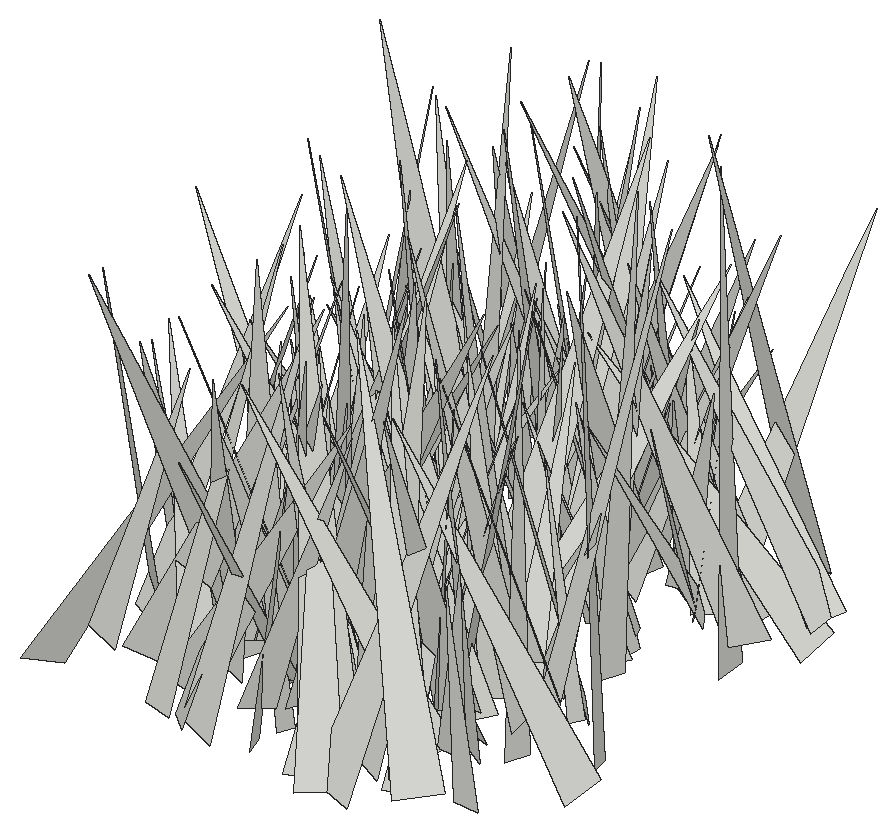
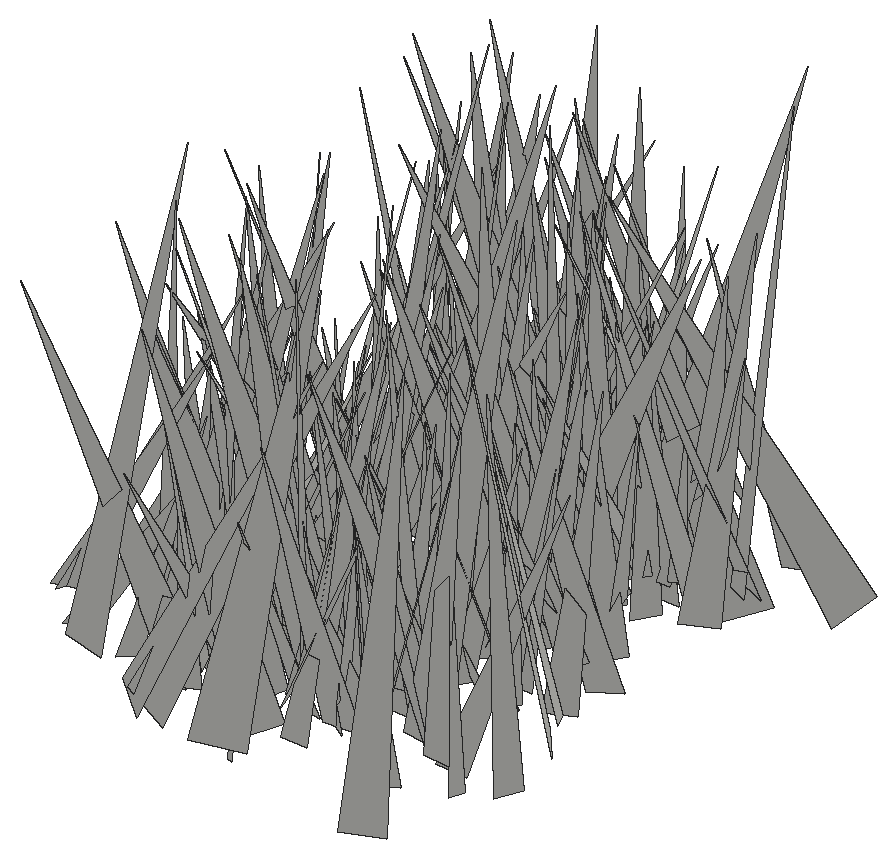
# SketchUp Ruby script. Lengths in inches.
U = 1.inch
M = Sketchup.active_model
def pt(a) = Geom::Point3d.new(a.map { |v| v * U })
def face(e, loops, mat)
  f = e.add_face(loops[0].map { |a| pt(a) })
  loops[1..].each { |l| e.add_face(l.map { |a| pt(a) }).erase! }
  f.material = f.back_material = mat if mat
  f
end
# faces: each face lists its corners as indices into pts; further lists are holes
def faces(e, pts, list, mat = nil) = list.each { |f| face(e, (f[0].is_a?(Array) ? f : [f]).map { |l| l.map { |i| pts[i] } }, mat) }
# xy, xz, yz: faces in a plane at the given z, y or x. An outline is a flat list of corners, or four numbers for a rectangle; further outlines are holes
def ring(l) = l.size == 4 ? [[l[0], l[1]], [l[2], l[1]], [l[2], l[3]], [l[0], l[3]]] : l.each_slice(2).to_a
def flat(e, list, mat, &to3) = list.each { |f| face(e, (f[0].is_a?(Array) ? f : [f]).map { |l| ring(l).map { |u, v| to3.(u, v) } }, mat) }
def xy(e, z, list, mat = nil) = flat(e, list, mat) { |x, y| [x, y, z] }
def xz(e, y, list, mat = nil) = flat(e, list, mat) { |x, z| [x, y, z] }
def yz(e, x, list, mat = nil) = flat(e, list, mat) { |y, z| [x, y, z] }
def lines(e, pts, list) = list.each { |a, b| e.add_line(pt(pts[a]), pt(pts[b])) }
# prism: a flat outline (further loops are holes) pulled along v
def prism(e, loops, v, mat = nil)
  f = face(e, loops, mat); d = Geom::Vector3d.new(v.map { |x| x * U })
  f.pushpull(f.normal.samedirection?(d) ? d.length : -d.length)
end
def box(e, o, s, mat = nil) = prism(e, [[o, [o[0] + s[0], o[1], o[2]], [o[0] + s[0], o[1] + s[1], o[2]], [o[0], o[1] + s[1], o[2]]]], [0, 0, s[2]], mat)
def at(x, y, z, deg = 0) = Geom::Transformation.translation(pt([x, y, z])) * Geom::Transformation.rotation(ORIGIN, Z_AXIS, deg.degrees)
def axes(o, x, y, z) = Geom::Transformation.new([*x, 0, *y, 0, *z, 0, *pt(o).to_a, 1])
def part(name) = M.definitions.add(name)
# library, detail: a bought-in or finely detailed component or shape, given as its bounding box
def library(name, o, s) = part(name).tap { |d| box(d.entities, o, s) }
def detail(e, o, s) = box(e.add_group.entities, o, s)
def put(e, d, t, mat = nil) = e.add_instance(d, t).tap { |i| i.material = mat if mat }
def group(e, t, mat = nil) = e.add_group.tap { |g| g.transformation = t; g.material = mat if mat }.entities
root = M.entities
c1 = part("fur_instance\#9")
p = [[0.8125,0,1.79],[0.67,-0.02,1.48],[0,-0.11,0],[0,0.11,0]]
faces(c1.entities,p,[[0,1,2,3]])
put(root,c1,axes([98.14,124.15,-28.22],[6.1777,-0.38175,1.16241],[-0.13775,-6.16226,-1.29169],[-1.21571,-1.24165,6.0532]))
put(root,c1,axes([98.83,114.34,-27.1],[4.29462,-4.11505,0.26594],[-3.98176,-4.23808,-1.27765],[-1.07236,-0.74374,5.80905]))
put(root,c1,axes([100.36,124.0625,-28.22],[1.56687,-4.2825,0.24372],[-4.04586,-1.5617,-1.43053],[-1.42486,-0.27491,4.32996]))
put(root,c1,axes([99.08,121,-28.22],[5.30824,4.83924,1.79848],[4.88732,-5.54151,0.48577],[-1.6634,-0.83881,7.16657]))
put(root,c1,axes([101.27,111.58,-28.22],[-5.02924,-0.94611,0.83871],[-1.10156,4.96734,-1.00192],[0.62059,1.14984,5.01842]))
put(root,c1,axes([99.2,112.08,-27.1],[-3.9717,-6.10655,1.7462],[-5.81347,4.32471,1.90107],[2.55787,0.34722,7.03209]))
put(root,c1,axes([101.37,114.98,-27.1],[-4.4304,-0.23548,0.66281],[-0.42328,4.26855,-1.31284],[0.56178,1.35914,4.23796]))
put(root,c1,axes([99.04,111.71,-27.1],[3.08355,6.47581,0.56476],[6.50039,-3.07095,-0.27862],[0.00972,-0.62967,7.16706]))
put(root,c1,axes([98.47,121.29,-27.1],[4.57096,2.53062,0.74602],[2.63797,-4.36083,-1.37058],[0.04077,-1.55993,5.04174]))
put(root,c1,axes([98.78,109.9,-27.1],[-0.11529,-4.79427,2.44231],[-5.06003,0.9271,1.58106],[1.8292,2.26244,4.52754]))
put(root,c1,axes([97.04,109.3,-28.22],[7.21653,-2.33327,0.39687],[-2.31249,-6.67999,2.77668],[0.50399,2.75925,7.05779]))
put(root,c1,axes([102.03,123.24,-28.22],[-1.21025,6.4146,1.42422],[6.45546,0.89059,1.47445],[-1.22575,-1.64315,6.35907]))
put(root,c1,axes([99.84,125.43,-27.1],[-1.49561,-5.63035,1.67127],[-5.71638,1.79132,0.91926],[1.34798,1.34949,5.75262]))
put(root,c1,axes([99.95,119.47,-28.22],[3.42227,-3.49613,0.30492],[-3.40506,-3.41104,-0.89344],[-0.84941,-0.41195,4.81005]))
put(root,c1,axes([101.46,111.12,-27.1],[-3.65531,3.57205,1.42816],[3.77376,3.712,0.37448],[0.74692,-1.27356,5.09712]))
put(root,c1,axes([99.32,125.1,-28.22],[4.97524,0.71585,1.07536],[1.04452,-4.74693,-1.67259],[-0.76015,-1.83742,4.74004]))
put(root,c1,axes([99.75,117.6,-28.22],[-0.68675,5.73435,1.62653],[5.78722,1.03346,-1.2],[1.42703,-1.4315,5.64928]))
put(root,c1,axes([101.83,119.48,-28.22],[4.02018,4.80904,4.066],[5.52928,-5.00439,0.45193],[-3.01434,-2.76593,6.25176]))
put(root,c1,axes([102.32,118.93,-28.22],[0.55965,-6.1533,3.26603],[-6.71098,-1.35523,-1.40332],[-1.86889,3.02383,6.01722]))
put(root,c1,axes([99.98,128.72,-28.22],[2.21636,-6.61774,0.25451],[-6.61771,-2.20273,0.35418],[0.25535,0.35358,6.97003]))
put(root,c1,axes([100.23,121.53,-27.1],[3.94789,-1.4658,0.35037],[-1.34081,-3.86465,-1.06014],[-0.68816,-0.87925,4.0756]))
put(root,c1,axes([102.05,125.84,-28.22],[-4.23671,-2.59002,0.97553],[-2.55905,4.34534,0.42292],[1.0541,0.13924,4.94763]))
put(root,c1,axes([99.33,113.69,-27.1],[6.39922,1.66084,0.77373],[1.68967,-6.43637,-0.15871],[-0.70856,-0.34898,6.60932]))
put(root,c1,axes([102.52,122.64,-27.1],[2.49125,-7.31611,3.2771],[-7.62751,-3.2193,-1.38865],[-2.46697,2.5655,7.60286]))
put(root,c1,axes([102.01,113.04,-27.1],[1.8393,-7.94223,0.20343],[-7.82957,-1.84746,-1.33722],[-1.34842,-0.10629,8.04201]))
put(root,c1,axes([104.88,114,-28.22],[-4.31341,6.46311,1.11663],[6.32564,3.74609,2.75266],[-1.73345,-2.41229,7.26637]))
put(root,c1,axes([101.51,119.68,-28.22],[2.15657,3.40289,0.33157],[3.29952,-2.17412,0.8525],[-0.89598,0.18416,3.93747]))
put(root,c1,axes([101.4,117.82,-27.1],[0.40052,6.46259,0.29319],[6.45769,-0.38185,-0.40475],[0.38629,-0.31712,6.46233]))
put(root,c1,axes([101.22,126,-28.22],[1.31397,-3.56018,1.31098],[-3.78942,-1.16427,0.63629],[0.18405,1.44556,3.7412]))
put(root,c1,axes([103.09,118.93,-27.1],[-4.66281,-2.88259,0.04543],[-2.761,4.48988,1.50703],[0.82963,-1.25893,5.27068]))
put(root,c1,axes([102.95,116.25,-27.1],[1.4221,-3.78822,2.5832],[-4.25079,-2.10312,-0.74405],[-1.71882,2.06693,3.97736]))
put(root,c1,axes([101.625,113.34,-28.22],[4.11916,-1.93041,1.42636],[-1.9279,-4.34864,-0.31782],[-1.42975,0.30221,4.53795]))
put(root,c1,axes([100.15,118.57,-27.1],[3.34433,-2.45993,0.06359],[-2.39384,-3.22746,1.0454],[0.56992,0.87868,4.01783]))
put(root,c1,axes([102.38,112.625,-27.1],[4.15865,3.49208,0.81847],[2.77358,-3.92559,2.6563],[-2.27416,1.59814,4.73636]))
put(root,c1,axes([103.42,119.94,-28.22],[-4.44101,1.77663,0.66677],[1.83519,4.45274,0.3588],[0.48276,-0.58331,4.76973]))
put(root,c1,axes([101.59,118.24,-27.1],[3.58428,-2.61771,1.24135],[-2.70899,-3.7283,-0.04015],[-1.02701,0.69843,4.43823]))
put(root,c1,axes([102.42,112.83,-27.1],[-3.32764,3.062,1.30373],[3.08153,3.53122,-0.42827],[1.25687,-0.55083,4.50173]))
put(root,c1,axes([100.88,116,-28.22],[4.9839,-2.53795,0.76874],[-2.53211,-5.04073,-0.2255],[-0.78777,0.14572,5.58834]))
put(root,c1,axes([102,123.35,-27.1],[-0.34341,4.80516,0.97397],[4.88667,0.41477,-0.32328],[0.39826,-0.94579,4.80656]))
put(root,c1,axes([101.98,122.5,-28.22],[7.12046,1.58475,2.39098],[0.70942,-7.17277,2.64146],[-2.77938,2.22916,6.79964]))
put(root,c1,axes([103.02,122.32,-27.1],[2.9733,6.47594,2.08154],[6.51847,-3.36189,1.14821],[-1.94427,-1.36785,7.03277]))
put(root,c1,axes([102.39,119.16,-27.1],[-3.17214,-2.54983,0.51656],[-2.07776,2.97317,1.9168],[1.56569,-1.22048,3.59026]))
put(root,c1,axes([101.21,112.8,-27.1],[0.94954,-6.1364,0.24208],[-6.03443,-0.88683,1.18943],[1.14,0.41683,6.09444]))
put(root,c1,axes([101.74,112.23,-28.22],[-1.04898,-5.12431,2.12616],[-5.35306,1.50327,0.98203],[1.45734,1.83333,5.13756]))
put(root,c1,axes([103.43,113.9,-27.1],[-4.06699,-5.2197,0.56162],[-5.13541,4.10303,0.94539],[1.09007,-0.14467,6.54919]))
put(root,c1,axes([99.42,111.39,-28.22],[4.40599,-6.63506,1.39046],[-6.52465,-3.70025,3.01783],[1.84021,2.76664,7.37085]))
put(root,c1,axes([102.875,113.8125,-28.22],[-5.47966,3.19166,2.7493],[3.39794,6.01513,-0.2105],[2.48986,-1.18473,6.33791]))
put(root,c1,axes([100.78,117.875,-27.1],[6.76067,1.19839,0.69108],[1.18973,-6.79585,0.14582],[-0.7059,0.02372,6.86451]))
put(root,c1,axes([102.77,107.54,-27.1],[3.19327,6.60837,0.52108],[6.51338,-3.23542,1.11669],[-1.23207,0.02336,7.254]))
put(root,c1,axes([102.13,125.58,-28.22],[1.67975,-3.93598,0.16611],[-3.93538,-1.66827,0.26597],[0.17974,0.25696,4.27115]))
put(root,c1,axes([104.22,118.83,-27.1],[-3.8782,-4.63911,2.52217],[-5.26639,3.62608,-1.42825],[0.38461,2.87286,5.87554]))
put(root,c1,axes([102.75,113.11,-28.22],[4.03542,0.28371,1.50858],[-0.2798,-4.0361,1.5075],[-1.50932,1.50677,3.754]))
put(root,c1,axes([105.63,125.09,-27.1],[-6.50715,-2.26194,0.29712],[-2.26712,6.51165,-0.07913],[0.25462,0.17236,6.88863]))
put(root,c1,axes([105.23,110.48,-28.22],[-5.59441,-0.96055,0.72122],[-1.15543,5.24244,-1.98041],[0.32833,2.08191,5.31959]))
put(root,c1,axes([102.46,108.91,-28.22],[4.99959,5.18328,0.38062],[5.01525,-4.9501,1.53324],[-1.36326,0.79826,7.03643]))
put(root,c1,axes([103.625,122.35,-28.22],[0.28904,-4.61969,1.68996],[-4.89331,-0.44312,-0.3744],[-0.50298,1.65624,4.61355]))
put(root,c1,axes([103.96,120.3,-28.22],[-2.34318,3.21724,1.23905],[3.43189,2.31946,0.46753],[0.3286,-1.2829,3.95253]))
put(root,c1,axes([105.48,115.31,-27.1],[-6.50951,0.22142,0.60358],[0.38251,6.26967,1.82536],[0.51674,-1.85181,6.25226]))
put(root,c1,axes([101.25,116.84,-27.1],[4.31446,-3.71791,0.40504],[-3.72385,-4.21342,0.9907],[0.3462,1.01276,5.60856]))
put(root,c1,axes([105.25,120.8,-28.22],[-3.16425,3.77948,0.90882],[3.82647,2.82214,1.58634],[-0.68447,-1.69527,4.66695]))
put(root,c1,axes([103.5,112.99,-27.1],[2.17041,-4.52553,0.56409],[-4.42394,-2.24099,-0.95709],[-1.10786,0.0828,4.92697]))
put(root,c1,axes([103.29,124.42,-28.22],[3.14318,2.78213,1.66083],[2.96777,-3.40061,0.07991],[-1.30037,-1.03624,4.19683]))
put(root,c1,axes([102.6,112.77,-27.1],[4.53182,-5.76132,1.66498],[-5.89155,-4.66684,-0.11276],[-1.12014,1.237,7.32923]))
put(root,c1,axes([102.74,115.75,-27.1],[3.92592,-0.41216,0.89749],[-0.2951,-4.00034,-0.54626],[-0.94248,-0.46433,3.90952]))
put(root,c1,axes([102.89,115.99,-27.1],[7.08469,1.17747,2.52447],[1.61288,-7.35894,-1.094],[-2.27113,-1.55299,7.09806]))
put(root,c1,axes([104.9,114.22,-27.1],[-2.89308,-3.13599,0.85003],[-3.23039,2.89836,-0.3018],[0.34876,0.83187,4.25597]))
put(root,c1,axes([104.75,111.4,-27.1],[-0.95692,-4.60949,0.0097],[-4.59629,0.95343,-0.35816],[-0.34872,0.08227,4.69412]))
put(root,c1,axes([104.39,124.12,-28.22],[-0.48607,6.36101,0.33267],[6.36907,0.48063,0.1158],[-0.09028,-0.34048,6.37851]))
put(root,c1,axes([105.125,125.07,-27.1],[-5.04486,-3.51647,1.75014],[-3.733,5.17856,-0.35556],[1.22196,1.30239,6.1392]))
put(root,c1,axes([103.22,108.76,-28.22],[2.79902,6.82497,1.56007],[7.00009,-2.70115,-0.74237],[0.11309,-1.72399,7.33919]))
put(root,c1,axes([104.97,117.08,-27.1],[4.62611,-3.05223,2.53258],[-2.97331,-5.24406,-0.88892],[-2.62479,0.5609,5.47054]))
put(root,c1,axes([104.53,115.29,-28.22],[-1.51621,-3.26203,0.55212],[-3.23761,1.58793,0.49084],[0.68086,0.28668,3.56354]))
put(root,c1,axes([105.04,125.63,-28.22],[-0.82021,3.34867,1.94688],[3.86928,0.61559,0.57127],[-0.18046,-2.02092,3.4]))
put(root,c1,axes([105.37,124.63,-27.1],[4.87258,-2.82126,2.84071],[-2.53321,-5.63755,-1.25383],[-3.10033,0.17232,5.48903]))
put(root,c1,axes([106.01,112.08,-28.22],[1.80379,6.11401,2.80003],[6.29213,-2.55743,1.53087],[-2.37284,-2.13386,6.18799]))
put(root,c1,axes([104.35,124.18,-27.1],[-6.11732,-3.75265,2.76683],[-3.28898,6.70851,1.82699],[3.3046,-0.26993,6.94018]))
put(root,c1,axes([106.53,121.54,-28.22],[-3.19994,-2.12817,0.10035],[-2.08753,3.09569,-0.91527],[-0.42587,0.81635,3.73243]))
put(root,c1,axes([102.64,116.68,-27.1],[3.58397,-3.64133,0.7361],[-3.60405,-3.15993,1.91614],[0.90107,1.84433,4.7363]))
put(root,c1,axes([102.43,119.9375,-28.22],[2.95433,4.07724,0.35212],[3.82019,-2.59183,-2.04072],[1.46767,-1.46099,4.60298]))
put(root,c1,axes([105.16,119.47,-28.22],[-3.94466,-0.14605,1.57067],[-0.23954,4.23653,-0.20765],[1.55915,0.28136,3.94189]))
put(root,c1,axes([102.15,113.34,-27.1],[0.44147,-7.17503,0.62576],[-6.54369,-0.13768,3.03788],[3.00878,0.75334,6.51516]))
put(root,c1,axes([101.4,110.5625,-28.22],[2.95462,-6.48005,1.02046],[-5.97059,-2.19282,3.36242],[2.71745,2.2277,6.27814]))
put(root,c1,axes([104.05,123.45,-28.22],[4.56042,0.58445,0.815],[0.35248,-4.48653,1.24501],[-0.93891,1.15443,4.42595]))
put(root,c1,axes([103.53,117.95,-28.22],[5.04429,-5.44094,0.7168],[-5.46997,-5.06343,0.05905],[-0.44381,0.56596,7.41924]))
put(root,c1,axes([108.02,115.52,-27.1],[-2.44299,5.49091,1.30941],[5.27932,1.71736,2.64808],[-1.99837,-2.17564,5.395]))
put(root,c1,axes([105.74,124.12,-28.22],[-6.60957,-3.13791,3.29203],[-3.79035,7.01015,-0.92809],[2.51341,2.31982,7.25752]))
put(root,c1,axes([105.08,109.2,-28.22],[3.80415,1.70942,1.42934],[1.7089,-4.05302,0.29902],[-1.42996,-0.29602,4.15984]))
put(root,c1,axes([105.375,128.8,-27.1],[3.52334,-7.25518,1.10129],[-7.15699,-3.66725,-1.26216],[-1.62106,0.42196,7.96608]))
put(root,c1,axes([103.17,113.27,-27.1],[-1.64763,-7.14584,1.34901],[-6.49832,2.06763,3.01567],[3.26416,0.50931,6.68457]))
put(root,c1,axes([104.97,112.11,-28.22],[2.23095,-4.80055,1.901],[-5.14348,-2.24733,0.36107],[-0.45138,1.8816,5.28129]))
put(root,c1,axes([107.02,121.95,-27.1],[0.33091,4.05955,1.18914],[3.81261,-0.80293,1.68011],[-1.83248,-0.93747,3.71034]))
put(root,c1,axes([104.64,122.92,-27.1],[4.0424,-1.6774,0.68877],[-1.67315,-4.09915,-0.16314],[-0.69903,0.11126,4.37357]))
put(root,c1,axes([106.53,111.62,-27.1],[-5.73495,-0.11109,1.68244],[-0.04447,5.97258,0.24275],[1.68552,-0.22038,5.73089]))
put(root,c1,axes([104.8,124.03,-28.22],[4.37398,5.97616,2.1686],[6.29129,-4.44766,-0.43255],[-0.91492,-2.01317,7.39318]))
put(root,c1,axes([105.84,123.94,-28.22],[0.66695,4.37993,0.08385],[4.36286,-0.67176,0.3871],[-0.39533,-0.02429,4.41347]))
put(root,c1,axes([105.49,122.68,-27.1],[4.4988,1.24272,1.44893],[1.33102,-4.70119,-0.10058],[-1.36826,-0.48722,4.6662]))
put(root,c1,axes([104.51,116.63,-27.1],[3.63193,-4.05591,1.60644],[-4.34601,-3.18259,1.79036],[0.37856,2.37544,5.14159]))
put(root,c1,axes([104.67,112.99,-27.1],[1.53942,-5.44162,0.89342],[-5.38829,-1.28703,1.44538],[1.17292,1.22946,5.46735]))
put(root,c1,axes([105.83,127.66,-28.22],[-2.04339,-2.88899,0.9747],[-2.5158,2.26047,1.42575],[1.7225,-0.12566,3.23866]))
put(root,c1,axes([105.66,114.1,-28.22],[4.8037,-2.51399,0.9877],[-2.43404,-4.90267,-0.64073],[-1.17095,-0.12226,5.38379]))
put(root,c1,axes([109.76,126.71,-28.22],[-2.49506,-7.82927,1.12782],[-7.54738,2.00233,-2.79687],[-2.3678,1.86761,7.7266]))
put(root,c1,axes([108.26,124.31,-27.1],[1.91991,5.69676,2.84026],[5.7974,-2.78995,1.67703],[-2.62873,-1.9923,5.77292]))
put(root,c1,axes([103.42,112.56,-28.22],[7.5928,-1.32868,0.07278],[-1.31152,-7.40102,1.71058],[0.22497,1.69728,7.51598]))
put(root,c1,axes([107.43,110.45,-28.22],[0.0044,-6.27087,2.13822],[-6.5778,-0.25997,-0.7489],[-0.79272,2.12236,6.226]))
put(root,c1,axes([107.67,109.45,-27.1],[-5.36752,5.77658,2.45123],[6.12108,5.53013,0.37117],[1.38195,-2.05828,7.87664]))
put(root,c1,axes([104.99,109.43,-27.1],[4.67154,-2.82363,0.84685],[-2.94301,-4.55853,1.0353],[-0.16964,1.32674,5.35951]))
put(root,c1,axes([108.83,114.6875,-27.1],[-7.81883,2.51294,1.68172],[2.76611,7.82758,1.16397],[1.22135,-1.64052,8.12983]))
put(root,c1,axes([106.93,113.53,-28.22],[4.42317,-1.03576,2.17466],[-1.28949,-4.85884,0.30856],[-2.03449,0.82776,4.53233]))
put(root,c1,axes([107.74,119.22,-27.1],[-4.70779,-0.34884,1.44292],[-0.70643,4.74641,-1.15738],[1.30563,1.3103,4.57662]))
put(root,c1,axes([108.62,123.5,-27.1],[-4.68733,-0.90911,0.30449],[-0.85582,4.65242,0.7161],[0.43216,-0.64711,4.72067]))
put(root,c1,axes([108.31,108.19,-28.22],[-4.20959,5.12778,0.85898],[5.1677,4.24809,-0.03415],[0.57165,-0.64206,6.63427]))
put(root,c1,axes([107.24,108.55,-28.22],[-3.3116,2.69695,0.72945],[2.42136,3.33487,-1.33716],[1.39378,0.61437,4.05614]))
put(root,c1,axes([107.44,121.69,-27.1],[-5.06165,5.7028,1.49455],[5.55918,5.27278,-1.292],[1.96243,-0.22764,7.51486]))
put(root,c1,axes([110.46,126.56,-28.22],[-4.44374,-5.75342,0.61079],[-5.6055,4.0905,-2.25122],[-1.43294,1.84058,6.91236]))
put(root,c1,axes([107.72,115.18,-27.1],[4.54557,4.08977,3.87164],[5.12111,-5.0718,-0.65499],[-2.34307,-3.15097,6.07942]))
put(root,c1,axes([106.4,121.34,-28.22],[5.27182,0.13194,1.25121],[0.40362,-5.28245,-1.14356],[-1.19165,-1.2055,5.14798]))
put(root,c1,axes([103.93,113.08,-27.1],[6.6749,-4.96789,0.00129],[-4.8195,-6.47499,2.02019],[1.20515,1.62135,8.07174]))
put(root,c1,axes([105.26,123.65,-27.1],[6.69732,-3.52244,1.21858],[-3.71872,-6.48437,1.69431],[-0.25228,2.07171,7.37503]))
put(root,c1,axes([105.97,110.68,-27.1],[7.40162,-2.04644,1.37858],[-2.14984,-7.48787,0.42713],[-1.21103,0.78507,7.66743]))
put(root,c1,axes([110.8,110.59,-27.1],[-6.49837,1.01991,0.13564],[1.01971,6.26851,1.71854],[-0.13717,-1.71841,6.34946]))
put(root,c1,axes([107.12,118.16,-27.1],[-0.59068,7.87895,1.19707],[7.83923,0.79048,-1.33468],[1.43434,-1.07565,7.78752]))
put(root,c1,axes([109.12,117.21,-28.22],[-5.83631,0.9789,1.84731],[1.28037,6.00401,0.86359],[1.65271,-1.19453,5.85448]))
put(root,c1,axes([107.23,121.77,-27.1],[6.03648,4.13261,1.07509],[4.02235,-6.12795,0.97074],[-1.43354,0.20766,7.25088]))
put(root,c1,axes([110.875,119.98,-27.1],[-4.67684,-2.75,0.36196],[-2.71074,4.38122,-1.73872],[-0.58771,1.67594,5.13928]))
put(root,c1,axes([110.32,119.79,-28.22],[-0.27177,-3.75184,1.87256],[-3.70908,-0.66019,-1.86105],[-1.95589,1.77327,3.26904]))
put(root,c1,axes([106.18,125.72,-28.22],[5.13759,-3.83835,0.8309],[-3.9202,-4.93031,1.46363],[0.23526,1.66651,6.24384]))
put(root,c1,axes([109.11,113.11,-28.22],[1.20703,6.81999,0.05967],[6.70849,-1.19813,1.23829],[-1.22962,0.158,6.81439]))
put(root,c1,axes([109.48,116.62,-27.1],[0.38107,-4.3176,1.24457],[-4.35966,-0.65774,-0.94692],[-1.08815,1.12319,4.22969]))
put(root,c1,axes([110.44,114.71,-27.1],[1.97558,6.78512,3.04566],[6.89111,-2.85534,1.89119],[-2.79761,-2.24188,6.80913]))
put(root,c1,axes([108.5,121.21,-28.22],[1.2889,-4.23263,0.01136],[-4.22076,-1.28617,-0.32791],[-0.31699,-0.08469,4.41236]))
put(root,c1,axes([110.48,113.01,-27.1],[-2.9134,4.03937,1.46912],[4.26943,2.51447,1.5531],[-0.49677,-2.07934,4.73205]))
put(root,c1,axes([107.1875,125.3125,-27.1],[3.6219,-1.04912,0.12415],[-1.02885,-3.40219,1.26523],[0.23987,1.24847,3.55218]))
put(root,c1,axes([109.625,113.74,-28.22],[-1.99035,-6.59495,0.1128],[-6.59501,1.99173,0.07994],[0.10913,0.08488,6.88828]))
put(root,c1,axes([108.77,118.82,-27.1],[1.7832,7.11152,0.69499],[7.11724,-1.83129,0.47737],[-0.63379,-0.55606,7.31612]))
put(root,c1,axes([108.33,111.11,-27.1],[4.86014,-4.74094,2.82615],[-5.30574,-5.05065,0.65171],[-1.52079,2.46963,6.75816]))
put(root,c1,axes([108.34,118.33,-28.22],[4.76717,4.34009,0.09976],[4.0907,-4.54047,2.05487],[-1.45344,1.45601,6.11063]))
put(root,c1,axes([109.58,124.45,-27.1],[-2.16653,-7.31637,0.90738],[-7.36569,2.18851,0.05952],[0.3151,0.85299,7.63018]))
put(root,c1,axes([108.58,111.3125,-27.1],[4.22042,3.02936,0.44277],[2.70703,-4.0447,1.87014],[-1.43005,1.2839,4.84681]))
put(root,c1,axes([107.79,122.09,-27.1],[3.74369,-0.67268,0.40161],[-0.71907,-3.7286,0.45768],[-0.31101,0.52348,3.776]))
put(root,c1,axes([109.47,116.25,-28.22],[-1.60174,4.9541,0.61833],[4.97114,1.64265,-0.28364],[0.46172,-0.4996,5.19887]))
put(root,c1,axes([107.3,123.88,-28.22],[5.75538,-1.33671,0.29214],[-1.31847,-5.75568,-0.36093],[-0.36579,-0.28603,5.89753]))
put(root,c1,axes([107.13,119.28,-28.22],[3.7363,2.07589,0.22504],[1.88074,-3.14536,-2.2112],[0.90706,-2.02911,3.65784]))
put(root,c1,axes([108.72,125.19,-27.1],[3.70099,1.78589,1.07617],[1.91017,-3.78303,-0.29128],[-0.83593,-0.7377,4.09901]))
put(root,c1,axes([108.59,110.14,-28.22],[2.68485,5.08236,0.90598],[5.15716,-2.6868,-0.21076],[-0.23424,-0.9002,5.74408]))
put(root,c1,axes([110.1,109.57,-28.22],[-3.90191,2.21296,0.38649],[1.88444,3.64598,-1.85127],[1.22289,1.44261,4.08594]))
put(root,c1,axes([111.21,108.85,-27.1],[-0.8728,6.82324,1.17968],[6.78553,0.6058,1.51645],[-1.38016,-1.33658,6.7096]))
put(root,c1,axes([108.84,122.55,-27.1],[5.9537,-4.05045,0.58701],[-3.75603,-5.81897,-2.05648],[-1.62572,-1.38951,6.90098]))
put(root,c1,axes([111.57,113.82,-27.1],[-7.78363,-1.77881,1.5879],[-1.77027,7.9428,0.22014],[1.59741,0.13482,7.98126]))
put(root,c1,axes([109.64,123.85,-28.22],[-3.27673,-6.38483,2.25273],[-6.55108,3.62196,0.73666],[1.71005,1.64109,7.13865]))
put(root,c1,axes([110.19,114.35,-27.1],[1.93856,-5.12728,2.24723],[-5.46022,-2.25638,-0.43794],[-1.23493,1.9279,5.46399]))
put(root,c1,axes([108.59,121.4,-27.1],[1.5633,5.69815,3.01797],[6.40687,-1.02237,-1.38843],[0.72737,-3.24142,5.74326]))
put(root,c1,axes([112.04,108.21,-27.1],[-4.84886,5.21937,0.60309],[5.25064,4.78392,0.8135],[-0.19034,-0.99462,7.07753]))
put(root,c1,axes([108.3125,117.06,-28.22],[-2.65177,6.66161,0.65253],[5.97681,2.67255,-2.995],[3.01341,0.56142,6.51452]))
put(root,c1,axes([108.25,113.45,-27.1],[4.56554,2.4835,0.72557],[2.58092,-4.47494,-0.92307],[-0.18188,-1.15993,5.11467]))
put(root,c1,axes([109.375,112.24,-28.22],[5.0794,2.90769,2.21904],[3.29641,-5.28463,-0.62087],[-1.58507,-1.67247,5.81975]))
put(root,c1,axes([109.44,125.01,-28.22],[0.85171,-3.4207,0.8533],[-3.50883,-0.73716,0.54719],[0.34265,0.95401,3.48241]))
put(root,c1,axes([110.32,125.18,-28.22],[1.25653,-6.81976,0.6894],[-6.81087,-1.32116,-0.65555],[-0.77223,0.55558,6.90349]))
put(root,c1,axes([108.59,108.31,-28.22],[1.72672,7.47142,1.23195],[7.48463,-1.49226,-1.44043],[1.14896,-1.50745,7.53186]))
put(root,c1,axes([109.79,112.9,-27.1],[2.0561,-6.44135,0.2848],[-6.4395,-2.06652,-0.24899],[-0.32395,0.19535,6.75697]))
put(root,c1,axes([110.26,120.1,-28.22],[4.51587,-1.82573,1.61231],[-1.49442,-4.75873,-1.20297],[-1.92343,-0.58918,4.72009]))
put(root,c1,axes([111.0625,115.85,-27.1],[-3.86726,-4.8383,0.71579],[-4.78645,3.93151,0.71436],[1.00566,0.10641,6.1526]))
put(root,c1,axes([111.6,113.41,-28.22],[-6.28866,-0.36775,1.68536],[-0.82762,6.23312,-1.72806],[1.51351,1.8804,6.05775]))
put(root,c1,axes([109.0625,121.74,-27.1],[2.45412,4.72767,0.6627],[4.74881,-2.3413,-0.8831],[0.48874,-0.99004,5.25297]))
put(root,c1,axes([111.41,116.9,-28.22],[-4.76298,-4.61729,1.21885],[-4.61962,4.89113,0.47635],[1.20999,0.49843,6.61653]))
put(root,c1,axes([109.79,112.85,-27.1],[6.18065,2.99725,1.89028],[2.99834,-6.44896,0.42186],[-1.88855,-0.42956,6.85609]))
put(root,c1,axes([108.24,123.4,-27.1],[6.2285,-2.9564,0.62521],[-3.02175,-6.08711,1.31964],[0.01382,1.46019,6.76705]))
put(root,c1,axes([111.72,111.18,-27.1],[-3.6941,-4.73944,2.34113],[-5.23892,3.66336,-0.85037],[0.70493,2.38895,5.94858]))
put(root,c1,axes([113.85,121.47,-27.1],[-2.36054,6.29762,2.85628],[6.53149,1.03928,3.10644],[-2.27111,-3.55673,5.96508]))
put(root,c1,axes([111.79,122.09,-27.1],[-2.18486,3.79279,1.02862],[3.92891,2.13324,0.47945],[0.08359,-1.13179,4.35074]))
put(root,c1,axes([111.93,117.32,-27.1],[-7.13651,-0.0123,2.39844],[-0.61978,7.28244,-1.80677],[2.31701,1.91008,6.90402]))
put(root,c1,axes([112.02,124.65,-28.22],[-3.89042,0.9571,1.21715],[1.27935,3.84105,1.06884],[0.87221,-1.36496,3.86121]))
put(root,c1,axes([114.32,124.09,-28.22],[-5.96221,1.49508,0.02596],[1.36332,5.39133,2.61894],[-0.61423,-2.54602,5.56097]))
put(root,c1,axes([112.8,114.67,-27.1],[-3.94683,-0.00707,0.27926],[-0.08275,3.80753,-1.07302],[0.26682,1.07619,3.79817]))
put(root,c1,axes([109.81,117.16,-28.22],[1.41621,-4.16021,0.5332],[-4.01988,-1.18575,1.42542],[1.19673,0.94019,4.15706]))
put(root,c1,axes([111.72,122.05,-27.1],[-3.93384,-2.91751,0.42121],[-2.51987,3.69278,2.04402],[1.52955,-1.41982,4.45073]))
put(root,c1,axes([111.57,121.73,-27.1],[-2.88957,-1.62735,2.00469],[-2.2228,3.09866,-0.68855],[1.31385,1.66334,3.24403]))
put(root,c1,axes([110.3,122.77,-27.1],[2.04033,-4.0488,0.48109],[-4.03745,-1.93127,0.8697],[0.56854,0.81522,4.44965]))
put(root,c1,axes([113.76,114.58,-28.22],[-7.32928,-2.99407,2.48715],[-3.76161,6.81126,-2.88543],[1.00033,3.67572,7.37273]))
put(root,c1,axes([112.21,126.55,-27.1],[-2.39726,-7.68863,1.50052],[-7.81274,2.46126,0.12966],[0.5725,1.39306,8.05265]))
put(root,c1,axes([114.41,112.98,-28.22],[-6.59727,0.97904,0.29915],[1.02311,6.37288,1.70633],[0.03533,-1.73199,6.44755]))
put(root,c1,axes([111.3,122.02,-27.1],[-2.16154,-4.08693,0.6496],[-3.73051,2.24163,1.68984],[1.79115,-0.26331,4.30345]))
put(root,c1,axes([114.72,124.03,-27.1],[-4.43376,3.47486,0.22998],[3.34427,4.14468,1.85019],[-0.97128,-1.59146,5.32068]))
put(root,c1,axes([113.21,121.39,-28.22],[-7.33304,-1.55705,2.53328],[-2.07568,7.50758,-1.39398],[2.1292,1.95633,7.36578]))
put(root,c1,axes([111.18,110.84,-27.1],[0.91273,-4.1627,0.50654],[-4.12867,-0.80133,0.85424],[0.734,0.66898,4.1751]))
put(root,c1,axes([114.79,123.91,-27.1],[-6.1435,0.43905,0.01492],[0.43419,6.03663,1.1429],[-0.06685,-1.14104,6.05221]))
put(root,c1,axes([110.62,123.92,-28.22],[-0.63507,6.95916,1.46669],[6.78735,1.03289,-1.962],[2.12438,-1.21968,6.70699]))
put(root,c1,axes([112.5625,113.3,-27.1],[3.79972,6.90357,0.39781],[6.61789,-3.76205,2.07507],[-2.00527,0.66563,7.60206]))
put(root,c1,axes([112.24,110.18,-28.22],[0.0054,-4.02258,1.09842],[-4.16704,0.03516,0.14925],[0.15324,1.09787,4.01982]))
